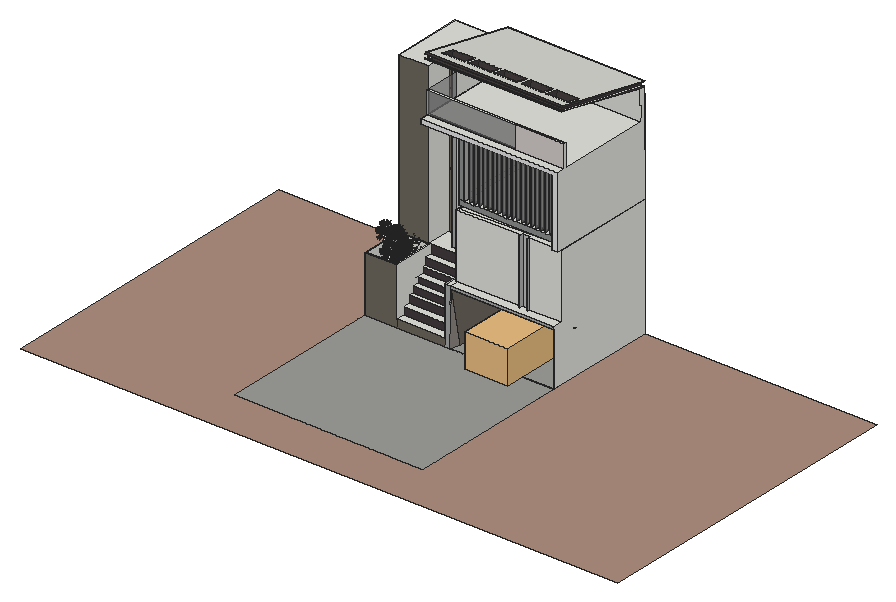
# SketchUp Ruby script. Lengths in inches.
U = 1.inch
M = Sketchup.active_model
def pt(a) = Geom::Point3d.new(a.map { |v| v * U })
def face(e, loops, mat)
  f = e.add_face(loops[0].map { |a| pt(a) })
  loops[1..].each { |l| e.add_face(l.map { |a| pt(a) }).erase! }
  f.material = f.back_material = mat if mat
  f
end
# faces: each face lists its corners as indices into pts; further lists are holes
def faces(e, pts, list, mat = nil) = list.each { |f| face(e, (f[0].is_a?(Array) ? f : [f]).map { |l| l.map { |i| pts[i] } }, mat) }
# xy, xz, yz: faces in a plane at the given z, y or x. An outline is a flat list of corners, or four numbers for a rectangle; further outlines are holes
def ring(l) = l.size == 4 ? [[l[0], l[1]], [l[2], l[1]], [l[2], l[3]], [l[0], l[3]]] : l.each_slice(2).to_a
def flat(e, list, mat, &to3) = list.each { |f| face(e, (f[0].is_a?(Array) ? f : [f]).map { |l| ring(l).map { |u, v| to3.(u, v) } }, mat) }
def xy(e, z, list, mat = nil) = flat(e, list, mat) { |x, y| [x, y, z] }
def xz(e, y, list, mat = nil) = flat(e, list, mat) { |x, z| [x, y, z] }
def yz(e, x, list, mat = nil) = flat(e, list, mat) { |y, z| [x, y, z] }
def lines(e, pts, list) = list.each { |a, b| e.add_line(pt(pts[a]), pt(pts[b])) }
# prism: a flat outline (further loops are holes) pulled along v
def prism(e, loops, v, mat = nil)
  f = face(e, loops, mat); d = Geom::Vector3d.new(v.map { |x| x * U })
  f.pushpull(f.normal.samedirection?(d) ? d.length : -d.length)
end
def box(e, o, s, mat = nil) = prism(e, [[o, [o[0] + s[0], o[1], o[2]], [o[0] + s[0], o[1] + s[1], o[2]], [o[0], o[1] + s[1], o[2]]]], [0, 0, s[2]], mat)
def at(x, y, z, deg = 0) = Geom::Transformation.translation(pt([x, y, z])) * Geom::Transformation.rotation(ORIGIN, Z_AXIS, deg.degrees)
def axes(o, x, y, z) = Geom::Transformation.new([*x, 0, *y, 0, *z, 0, *pt(o).to_a, 1])
def part(name) = M.definitions.add(name)
# library, detail: a bought-in or finely detailed component or shape, given as its bounding box
def library(name, o, s) = part(name).tap { |d| box(d.entities, o, s) }
def detail(e, o, s) = box(e.add_group.entities, o, s)
def put(e, d, t, mat = nil) = e.add_instance(d, t).tap { |i| i.material = mat if mat }
def group(e, t, mat = nil) = e.add_group.tap { |g| g.transformation = t; g.material = mat if mat }.entities
root = M.entities
M.materials.add("[Aluminum]").color = [179, 179, 179]
M.materials.add("[Asphalt New]").color = [67, 60, 62]
M.materials.add("[Blacktop Old 02]").color = [143, 145, 145]
M.materials.add("[Cladding Weathered]").color = [111, 105, 96]
M.materials.add("[Color M00]").color = [255, 255, 255]
M.materials.add("[Concrete Block 8x8 Gray]").color = [157, 158, 154]
M.materials.add("[Concrete Form 4x8]").color = [167, 170, 168]
M.materials.add("[Concrete Scored Jointless]").color = [140, 133, 127]
M.materials.add("[Metal Corrugated Shiny]").color = [193, 193, 193]
M.materials.add("[Pavers Modular Brick]").color = [175, 143, 129]
M.materials.add("[Polished Concrete Old]").color = [229, 229, 229]
M.materials.add("[Tile Hexagon White]").color = [213, 206, 204]
M.materials.add("[Translucent Glass Gray]").color = [128, 128, 128]
M.materials["[Translucent Glass Gray]"].alpha = 0.5
c1 = part("Group\#1")
xy(c1.entities,0,[[0.75,0,0.75,11.8125,1.49,9.04]])
p = [[0.75,11.8125,0],[0,8.59,0.28],[0.75,0,0]]
faces(c1.entities,p,[[0,1,2]])
c2 = part("Group\#2")
put(c2.entities,c1,axes([14.375,5.39,3.77],[0.45748,0.87256,0.17132],[-0.80767,0.48834,-0.33043],[-0.37199,0.0128,0.92815]))
put(c2.entities,c1,axes([-0.67,1.875,2.66],[0.89879,-0.42343,0.11346],[0.43837,0.86817,-0.23263],[0,0.25882,0.96593]))
put(c2.entities,c1,at(4.43,0,0))
c3 = part("Group\#11")
put(c3.entities,c2,axes([22.24,16.83,2.07],[-0.74431,0.66783,0],[-0.65748,-0.73278,-0.17537],[-0.11712,-0.13053,0.9845]))
put(c3.entities,c2,axes([5.44,0,2.07],[1,0,0],[0,0.9845,-0.17537],[0,0.17537,0.9845]))
put(c3.entities,c2,axes([11.93,24.29,2.07],[-0.95052,-0.31068,0],[0.30586,-0.93579,-0.17537],[0.05448,-0.16669,0.9845]))
c4 = part("Group\#4")
put(c4.entities,c3,axes([14.86,-1.73,0.2],[0.445,0.77076,0],[-0.77076,0.445,0],[0,0,1.5842]))
put(c4.entities,c3,at(0,0,0))
c5 = part("Group\#3")
put(c5.entities,c2,axes([22.24,16.83,2.07],[-0.74431,0.66783,0],[-0.65748,-0.73278,-0.17537],[-0.11712,-0.13053,0.9845]))
put(c5.entities,c2,axes([5.44,0,2.07],[1,0,0],[0,0.9845,-0.17537],[0,0.17537,0.9845]))
put(c5.entities,c2,axes([11.93,24.29,2.07],[-0.95052,-0.31068,0],[0.30586,-0.93579,-0.17537],[0.05448,-0.16669,0.9845]))
c6 = part("plant+06")
g1 = group(c6.entities,at(-18.2,-4.83,0,-28.132))
g2 = group(g1,at(16.21,1.96,0.15,45))
g3 = group(g2,at(0,13.2,6.74))
p = [[6.87,-6.88,6.35],[6.87,-6.88,1.06]]
lines(g3,p,[[0,1]])
put(g3,c3,axes([13.75,-0.59,5.87],[0,-0.5917,0],[-0.5917,0,0],[0,0,0.5917]))
put(g3,c3,axes([16.18,-7.3,4.96],[-0.4184,-0.4184,0],[-0.4184,0.4184,0],[0,0,0.39243]))
put(g3,c3,axes([7.21,-16.1875,5.36],[-0.45127,0.38271,0],[0.38271,0.45127,0],[0,0,0.5917]))
put(g3,c3,axes([9.38,1.03,7.16],[0.26331,-0.45606,0],[-0.45606,-0.26331,0],[0,0,0.93737]))
put(g3,c4,axes([11.69,-2.37,6.35],[0,-0.4246,0],[-0.41463,0,0],[0,0,0.79418]))
put(g3,c4,axes([13.04,-1.11,5.01],[0,-0.54349,0],[-0.53072,0,0],[0,0,-0.63534]))
g4 = group(g2,at(6.41,6.51,0))
yz(g4,0,[[2.84,0,3.35,0,3.59,0.57,3.4,0.57,3.35,1.6,2.95,3.43,2.26,4.68,1.45,5.78,0.57,8.92,0.06,13.45,0,8.85,0.92,5.52,1.78,4.37,2.41,3.22,2.78,1.53]])
g5 = group(g1,at(11.08,10.15,0))
p = [[0.67,0.67,15.45],[0.64,0.64,18.83],[1.01,1.01,27.22],[0.53,0.53,32.8],[0.79,0.79,27.32],[0.38,0.38,23.38],
  [0,0,18.98],[0.02,0.02,15.18],[1.0625,1.0625,8.07],[2,2,4.77],[2.6875,2.6875,0],[3.37,3.37,0],
  [3.15,3.15,1.52],[2.58,2.58,5.45],[1.65,1.65,8.75]]
faces(g5,p,[[0,1,2,3,4,5,6,7,8,9,10,11,12,13,14]])
g6 = group(g1,at(0,22.3,24.33))
p = [[11.61,-11.625,10.73],[11.61,-11.625,1.79]]
lines(g6,p,[[0,1]])
put(g6,c3,axes([23.24,-1,9.91],[0,-1,0],[-1,0,0],[0,0,1]))
put(g6,c3,axes([27.34,-12.34,8.39],[-0.70711,-0.70711,0],[-0.70711,0.70711,0],[0,0,0.66323]))
put(g6,c3,axes([12.1875,-27.36,9.06],[-0.76267,0.64679,0],[0.64679,0.76267,0],[0,0,1]))
put(g6,c5,axes([12.75,-8.02,11.21],[0.12015,-0.20811,0],[-0.20811,-0.12015,0],[0,0,2.51293]))
put(g6,c4,axes([19.76,-4,10.73],[0,-0.7176,0],[-0.70074,0,0],[0,0,1.3422]))
put(g6,c4,axes([22.04,-1.87,8.47],[0,-0.91853,0],[-0.89694,0,0],[0,0,-1.07376]))
g7 = group(g1,at(13.77,10.12,0.15))
yz(g7,0,[[3.35,0,3.86,0,5.625,2.125,6.92,4.34,7.79,6.82,9.06,9.4,9.5,10.42,9.57,11.59,9.18,14.18,9.77,19.63,8.6,14.17,8.89,11.53,8.79,10.51,8.36,9.61,6.96,7.04,6.47,5.81,6.17,4.6,5.15,2.46,3.59,0.57]])
g8 = group(g1,at(2.16,8.02,10.39))
p = [[11.61,11.625,10.73],[11.61,11.625,1.79]]
lines(g8,p,[[0,1]])
put(g8,c3,at(23.24,1,9.91,90))
put(g8,c3,axes([27.34,12.34,8.39],[-0.70711,0.70711,0],[-0.70711,-0.70711,0],[0,0,0.66323]))
put(g8,c3,at(12.1875,27.36,9.06,-139.7))
put(g8,c3,axes([15.85,-1.74,10.73],[0.445,0.77076,0],[-0.77076,0.445,0],[0,0,1.5842]))
put(g8,c4,axes([22.04,1.87,8.47],[0,0.91853,0],[-0.89694,0,0],[0,0,-1.07376]))
put(g8,c5,axes([12.75,15.23,10.63],[0.12015,-0.20811,0],[-0.20811,-0.12015,0],[0,0,2.11086]))
c7 = library("car\#1",[0.01,0.03,0.02],[18.76,39.97,12.32])
xy(root,0,[[256.5,66.7,532,304.75],[256.5,304.75,532,469.75]],"[Concrete Block 8x8 Gray]")
xy(root,0,[[0,0,0,469.75,256.5,469.75,256.5,66.7,532,66.7,532,469.75,868.5,469.75,868.5,0]],"[Pavers Modular Brick]")
xy(root,11.4375,[[303.32,304.75,373.81,317.05]])
xy(root,21.9375,[[303.32,317.05,373.81,327.17]])
xy(root,32.4375,[[303.32,327.17,373.81,333.97]])
xy(root,41.28,[[303.32,333.97,373.81,342.22]])
xy(root,50.125,[[303.32,342.22,373.81,352.48]])
xy(root,58.5625,[[303.32,352.48,373.81,356.36]])
xy(root,68.875,[[303.32,356.36,373.81,367.35]])
xy(root,77.99,[[383.9,304.75,528.81,468.375]],"[Concrete Scored Jointless]")
xy(root,81.1875,[[[256.5,304.75,303.32,367.35],[258.53,306.78,301.29,365.32]],[373.81,304.75,380.71,304.75,380.71,318.49,378.74,318.49,378.74,423.52,373.81,423.52],[380.71,304.75,532,304.75,532,318.49,484.37,318.49,484.37,315.8,483.53,315.8,483.53,320.92,473.54,320.92,473.54,315.8,472.125,315.8,472.125,318.49,380.71,318.49],[378.74,318.49,380.71,423.52],[299.38,367.35,373.81,367.35,373.81,423.52,332.89,423.52,332.89,377.29,325.25,377.29,325.25,403.55,299.38,403.55],
  [332.89,427.84,378.74,469.75]])
xy(root,103.5,[[336.62,423.34,338.18,427.84]],"[Translucent Glass Gray]")
xy(root,154.875,[[336.62,423.34,338.18,427.84]],"[Translucent Glass Gray]")
xy(root,174.1875,[[472.125,315.8,473.54,315.8,473.54,320.92,483.53,320.92,483.53,315.8,484.37,315.8,484.37,318.49,523.01,318.49,523.01,469.75,378.74,469.75,378.74,394.12,380.74,394.12,380.74,323.56,378.74,323.56,378.74,318.49,472.125,318.49],[523.01,318.49,532,469.75],[378.74,323.56,380.74,394.12]])
xy(root,175.74,[[523.01,311.36,532,469.75]])
xy(root,178.55,[[379.42,321.87,523.01,469.75]])
xy(root,186.36,[[387.1,321.87,388.32,328.37],[389.15,321.87,395.2,328.37],[396.02,321.87,402.07,328.37],[402.9,321.87,408.95,328.37],[409.77,321.87,415.82,328.37],
  [416.65,321.87,422.7,328.37],[423.52,321.87,429.57,328.37],[430.4,321.87,436.45,328.37],[437.27,321.87,443.32,328.37],[444.15,321.87,450.2,328.37],
  [451.02,321.87,457.07,328.37],[457.9,321.87,463.95,328.37],[464.77,321.87,470.82,328.37],[471.65,321.87,477.7,328.37],[478.52,321.87,484.57,328.37],
  [485.4,321.87,491.45,328.37],[492.27,321.87,498.32,328.37],[499.15,321.87,505.2,328.37],[506.02,321.87,512.07,328.37],[512.9,321.87,518.95,328.37],
  [519.77,321.87,523.01,328.37]])
xy(root,269.125,[[332.89,423.52,378.74,427.84]])
xy(root,270.4375,[[379.42,321.87,387.1,321.87,387.1,328.37,523.01,328.37,523.01,469.75,379.42,469.75],[388.32,321.87,389.15,328.37],[395.2,321.87,396.02,328.37],[402.07,321.87,402.9,328.37],[408.95,321.87,409.77,328.37],
  [415.82,321.87,416.65,328.37],[422.7,321.87,423.52,328.37],[429.57,321.87,430.4,328.37],[436.45,321.87,437.27,328.37],[443.32,321.87,444.15,328.37],
  [450.2,321.87,451.02,328.37],[457.07,321.87,457.9,328.37],[463.95,321.87,464.77,328.37],[470.82,321.87,471.65,328.37],[477.7,321.87,478.52,328.37],
  [484.57,321.87,485.4,328.37],[491.45,321.87,492.27,328.37],[498.32,321.87,499.15,328.37],[505.2,321.87,506.02,328.37],[512.07,321.87,512.9,328.37],
  [518.95,321.87,519.77,328.37]])
xy(root,272.72,[[332.89,311.36,523.01,469.75]])
xy(root,279.5,[[332.89,311.36,532,322.79],[332.89,325.46,532,461.81]])
xy(root,311.875,[[332.89,322.79,461.48,325.46],[461.48,322.79,532,325.46],[256.5,367.35,299.38,367.35,299.38,403.55,303.32,403.55,303.32,469.75,256.5,469.75],[325.25,377.29,332.89,469.75],[303.32,403.55,325.25,469.75]])
xy(root,323.37,[[332.89,467.54,339.64,467.82]])
xz(root,304.75,[[256.5,0,303.32,81.1875],[303.32,0,373.81,11.4375]],"[Cladding Weathered]")
xz(root,304.75,[[373.81,0,380.71,81.1875],[380.71,0,383.9,77.99,528.81,77.99,532,81.1875,380.71,81.1875]],"[Concrete Form 4x8]")
xz(root,306.78,[[258.53,63.625,301.29,81.1875]])
xz(root,311.36,[[523.01,175.74,532,175.74,532,279.5,332.89,279.5,332.89,272.72,523.01,272.72]],"[Polished Concrete Old]")
xz(root,315.8,[[472.125,81.1875,473.54,174.1875],[483.53,81.1875,484.37,174.1875]],"[Aluminum]")
xz(root,317.05,[[303.32,11.4375,373.81,21.9375]],"[Asphalt New]")
xz(root,318.42,[[332.89,354.89,532,356.22]],"[Asphalt New]")
xz(root,318.49,[[378.74,81.1875,472.125,174.1875],[484.37,81.1875,532,174.1875]])
xz(root,320.92,[[473.54,81.1875,483.53,174.1875]],"[Metal Corrugated Shiny]")
xz(root,321.87,[[379.42,178.55,523.01,178.55,523.01,186.36,519.77,186.36,519.77,270.4375,518.95,270.4375,518.95,186.36,512.9,186.36,512.9,270.4375,512.07,270.4375,512.07,186.36,506.02,186.36,506.02,270.4375,505.2,270.4375,505.2,186.36,499.15,186.36,499.15,270.4375,498.32,270.4375,498.32,186.36,492.27,186.36,492.27,270.4375,491.45,270.4375,491.45,186.36,485.4,186.36,485.4,270.4375,484.57,270.4375,484.57,186.36,478.52,186.36,478.52,270.4375,477.7,270.4375,477.7,186.36,471.65,186.36,471.65,270.4375,470.82,270.4375,470.82,186.36,464.77,186.36,464.77,270.4375,463.95,270.4375,463.95,186.36,457.9,186.36,457.9,270.4375,457.07,270.4375,457.07,186.36,451.02,186.36,451.02,270.4375,450.2,270.4375,450.2,186.36,444.15,186.36,444.15,270.4375,443.32,270.4375,443.32,186.36,437.27,186.36,437.27,270.4375,436.45,270.4375,436.45,186.36,430.4,186.36,430.4,270.4375,429.57,270.4375,429.57,186.36,423.52,186.36,423.52,270.4375,422.7,270.4375,422.7,186.36,416.65,186.36,416.65,270.4375,415.82,270.4375,415.82,186.36,409.77,186.36,409.77,270.4375,408.95,270.4375,408.95,186.36,402.9,186.36,402.9,270.4375,402.07,270.4375,402.07,186.36,396.02,186.36,396.02,270.4375,395.2,270.4375,395.2,186.36,389.15,186.36,389.15,270.4375,388.32,270.4375,388.32,186.36,379.42,186.36],[379.42,186.36,387.1,270.4375]],"[Blacktop Old 02]")
xz(root,322.79,[[461.48,279.5,532,311.875]],"[Tile Hexagon White]")
xz(root,322.79,[[332.89,279.5,461.48,311.875]],"[Translucent Glass Gray]")
xz(root,325.46,[[461.48,279.5,532,311.875]])
xz(root,325.46,[[332.89,279.5,461.48,311.875]],"[Translucent Glass Gray]")
xz(root,327.17,[[303.32,21.9375,373.81,32.4375]],"[Asphalt New]")
xz(root,328.37,[[387.1,186.36,388.32,270.4375]])
xz(root,328.37,[[389.15,186.36,395.2,270.4375],[396.02,186.36,402.07,270.4375],[402.9,186.36,408.95,270.4375],[409.77,186.36,415.82,270.4375],[416.65,186.36,422.7,270.4375],
  [423.52,186.36,429.57,270.4375],[430.4,186.36,436.45,270.4375],[437.27,186.36,443.32,270.4375],[444.15,186.36,450.2,270.4375],[451.02,186.36,457.07,270.4375],
  [457.9,186.36,463.95,270.4375],[464.77,186.36,470.82,270.4375],[471.65,186.36,477.7,270.4375],[478.52,186.36,484.57,270.4375],[485.4,186.36,491.45,270.4375],
  [492.27,186.36,498.32,270.4375],[499.15,186.36,505.2,270.4375],[506.02,186.36,512.07,270.4375],[512.9,186.36,518.95,270.4375],[519.77,186.36,523.01,270.4375]],"[Translucent Glass Gray]")
xz(root,333.97,[[303.32,32.4375,373.81,41.28]],"[Asphalt New]")
xz(root,342.22,[[303.32,41.28,373.81,50.125]],"[Asphalt New]")
xz(root,352.48,[[303.32,50.125,373.81,58.5625]],"[Asphalt New]")
xz(root,356.36,[[303.32,58.5625,373.81,68.875]],"[Asphalt New]")
xz(root,365.32,[[258.53,63.625,299.38,81.1875]])
xz(root,367.35,[[303.32,68.875,373.81,81.1875]],"[Asphalt New]")
xz(root,367.35,[[256.5,81.1875,299.38,311.875]],"[Cladding Weathered]")
xz(root,377.29,[[325.25,81.1875,332.89,311.875]],"[Concrete Form 4x8]")
xz(root,403.55,[[[302.32,122.77,325.25,299.71],[303.625,124.08,323.94,298.4]],[303.625,163.67,323.94,165.07],[303.625,219.03,323.94,220.97],[303.625,268.56,323.94,270.61]],"[Asphalt New]")
xz(root,403.55,[[299.38,81.1875,325.25,81.1875,325.25,122.77,302.32,122.77,302.32,299.71,325.25,299.71,325.25,311.875,299.38,311.875]],"[Cladding Weathered]")
xz(root,423.34,[[336.62,103.5,338.18,154.875]],"[Translucent Glass Gray]")
xz(root,423.52,[[332.89,177.19,378.74,180.2]],"[Asphalt New]")
xz(root,423.52,[[332.89,81.1875,378.74,177.19]],"[Translucent Glass Gray]")
xz(root,427.84,[[[332.89,81.1875,378.74,269.125],[336.62,103.5,338.18,154.875]]],"[Translucent Glass Gray]")
xz(root,468.375,[[383.9,3.19,528.81,77.99]],"[Cladding Weathered]")
xz(root,469.75,[[332.89,81.1875,378.74,272.72],[378.74,174.1875,378.74,272.72,523.01,272.72,523.01,270.4375,379.42,270.4375,379.42,178.55,380.74,178.55,380.74,174.1875],[380.74,174.1875,523.01,178.55],[523.01,174.1875,532,175.74],[523.01,175.74,523.01,178.55,379.42,178.55,379.42,270.4375,523.01,270.4375,523.01,182.6875,532,182.6875,532,175.74],
  [532,182.6875,523.01,270.4375,523.01,272.72,332.89,311.875,532,311.875],[523.01,182.6875,523.01,270.4375,532,182.6875],[332.89,272.72,332.89,311.875,523.01,272.72]])
xz(root,469.75,[[256.5,0,332.89,311.875],[332.89,0,332.89,81.1875,378.74,81.1875,378.74,174.1875,532,174.1875,532,0]],"[Color M00]")
yz(root,256.5,[[304.75,0,304.75,81.1875,367.35,81.1875,367.35,311.875,469.75,311.875,469.75,0]])
yz(root,258.53,[[306.78,63.625,365.32,81.1875]])
yz(root,299.38,[[367.35,81.1875,403.55,311.875]])
yz(root,303.32,[[304.75,11.4375,317.05,11.4375,317.05,21.9375,327.17,21.9375,327.17,32.4375,333.97,32.4375,333.97,41.28,342.22,41.28,342.22,50.125,352.48,50.125,352.48,58.5625,356.36,58.5625,356.36,68.875,367.35,68.875,367.35,81.1875,304.75,81.1875]])
yz(root,325.25,[[377.29,81.1875,403.55,311.875]])
yz(root,332.89,[[377.29,81.1875,423.52,81.1875,423.52,269.125,427.84,269.125,427.84,81.1875,469.75,81.1875,469.75,272.72,377.29,272.72],[311.36,272.72,377.29,279.5],[377.29,272.72,377.29,279.5,461.81,279.5,461.81,311.875,469.75,311.875,469.75,272.72],[322.79,279.5,325.46,311.875],[377.29,279.5,461.81,279.5,460.34,311.875,377.29,311.875],
  [461.81,279.5,461.81,311.875,460.34,311.875],[460.34,311.875,459.79,323.81,461.81,311.875],[461.81,311.875,459.79,323.81,467.54,322.11,469.75,311.875]])
yz(root,332.89,[[467.54,322.11,459.79,323.81,323.42,353.79,323.6875,355,467.54,323.37,467.82,323.37],[468.8,327.8125,324.68,359.5,319.67,360.6,320.06,362.35,469.18,329.5625]],"[Asphalt New]")
yz(root,332.89,[[325.46,279.5,377.29,311.875]],"[Translucent Glass Gray]")
yz(root,336.62,[[423.34,103.5,427.84,154.875]],"[Translucent Glass Gray]")
yz(root,338.18,[[423.34,103.5,427.84,154.875]],"[Translucent Glass Gray]")
yz(root,339.64,[[467.54,323.37,323.6875,355,324.68,359.5,468.8,327.8125,467.82,323.37]],"[Asphalt New]")
yz(root,344.65,[[353.31,347.22,354.95,354.68,335.23,359.01,333.59,351.56]],"[Asphalt New]")
yz(root,373.81,[[304.75,11.4375,304.75,81.1875,367.35,81.1875,367.35,68.875,356.36,68.875,356.36,58.5625,352.48,58.5625,352.48,50.125,342.22,50.125,342.22,41.28,333.97,41.28,333.97,32.4375,327.17,32.4375,327.17,21.9375,317.05,21.9375,317.05,11.4375]])
yz(root,377.31,[[353.31,347.22,333.59,351.56,335.23,359.01,354.95,354.68]])
yz(root,378.74,[[318.49,81.1875,423.52,174.1875],[427.84,81.1875,469.75,174.1875],[423.52,174.1875,427.84,269.125]])
yz(root,379.42,[[321.87,178.55,469.75,186.36],[321.87,186.36,469.75,270.4375]])
yz(root,382.28,[[353.31,347.22,354.95,354.68,335.23,359.01,333.59,351.56]],"[Asphalt New]")
yz(root,383.9,[[322.9,-14.85,468.375,3.19,468.375,77.99,304.75,77.99,468.375,3.82],[322.9,-14.85,468.375,3.82,304.75,77.99]],"[Cladding Weathered]")
yz(root,387.1,[[321.87,186.36,328.37,270.4375]])
yz(root,388.32,[[321.87,186.36,328.37,270.4375]])
yz(root,389.15,[[321.87,186.36,328.37,270.4375]],"[Translucent Glass Gray]")
yz(root,395.2,[[321.87,186.36,328.37,270.4375]],"[Translucent Glass Gray]")
yz(root,396.02,[[321.87,186.36,328.37,270.4375]],"[Translucent Glass Gray]")
yz(root,402.07,[[321.87,186.36,328.37,270.4375]],"[Translucent Glass Gray]")
yz(root,402.9,[[321.87,186.36,328.37,270.4375]],"[Translucent Glass Gray]")
yz(root,408.95,[[321.87,186.36,328.37,270.4375]],"[Translucent Glass Gray]")
yz(root,409.77,[[321.87,186.36,328.37,270.4375]],"[Translucent Glass Gray]")
yz(root,414.94,[[353.31,347.22,333.59,351.56,335.23,359.01,354.95,354.68]])
yz(root,415.82,[[321.87,186.36,328.37,270.4375]],"[Translucent Glass Gray]")
yz(root,416.65,[[321.87,186.36,328.37,270.4375]],"[Translucent Glass Gray]")
yz(root,420.09,[[353.31,347.22,354.95,354.68,335.23,359.01,333.59,351.56]],"[Asphalt New]")
yz(root,422.7,[[321.87,186.36,328.37,270.4375]],"[Translucent Glass Gray]")
yz(root,423.52,[[321.87,186.36,328.37,270.4375]],"[Translucent Glass Gray]")
yz(root,429.57,[[321.87,186.36,328.37,270.4375]],"[Translucent Glass Gray]")
yz(root,430.4,[[321.87,186.36,328.37,270.4375]],"[Translucent Glass Gray]")
yz(root,436.45,[[321.87,186.36,328.37,270.4375]],"[Translucent Glass Gray]")
yz(root,437.27,[[321.87,186.36,328.37,270.4375]],"[Translucent Glass Gray]")
yz(root,443.32,[[321.87,186.36,328.37,270.4375]],"[Translucent Glass Gray]")
yz(root,444.15,[[321.87,186.36,328.37,270.4375]],"[Translucent Glass Gray]")
yz(root,450.2,[[321.87,186.36,328.37,270.4375]],"[Translucent Glass Gray]")
yz(root,451.02,[[321.87,186.36,328.37,270.4375]],"[Translucent Glass Gray]")
yz(root,452.75,[[353.31,347.22,333.59,351.56,335.23,359.01,354.95,354.68]])
yz(root,457.07,[[321.87,186.36,328.37,270.4375]],"[Translucent Glass Gray]")
yz(root,457.9,[[321.87,186.36,328.37,270.4375]],"[Translucent Glass Gray]")
yz(root,458.15,[[353.31,347.22,354.95,354.68,335.23,359.01,333.59,351.56]],"[Asphalt New]")
yz(root,463.95,[[321.87,186.36,328.37,270.4375]],"[Translucent Glass Gray]")
yz(root,464.77,[[321.87,186.36,328.37,270.4375]],"[Translucent Glass Gray]")
yz(root,470.82,[[321.87,186.36,328.37,270.4375]],"[Translucent Glass Gray]")
yz(root,471.65,[[321.87,186.36,328.37,270.4375]],"[Translucent Glass Gray]")
yz(root,472.125,[[315.8,81.1875,318.49,174.1875]],"[Aluminum]")
yz(root,473.54,[[315.8,81.1875,320.92,174.1875]],"[Aluminum]")
yz(root,477.7,[[321.87,186.36,328.37,270.4375]],"[Translucent Glass Gray]")
yz(root,478.52,[[321.87,186.36,328.37,270.4375]],"[Translucent Glass Gray]")
yz(root,483.53,[[315.8,81.1875,320.92,174.1875]],"[Aluminum]")
yz(root,484.37,[[315.8,81.1875,318.49,174.1875]],"[Aluminum]")
yz(root,484.57,[[321.87,186.36,328.37,270.4375]],"[Translucent Glass Gray]")
yz(root,485.4,[[321.87,186.36,328.37,270.4375]],"[Translucent Glass Gray]")
yz(root,490.81,[[353.31,347.22,333.59,351.56,335.23,359.01,354.95,354.68]])
yz(root,491.45,[[321.87,186.36,328.37,270.4375]],"[Translucent Glass Gray]")
yz(root,492.27,[[321.87,186.36,328.37,270.4375]],"[Translucent Glass Gray]")
yz(root,495.65,[[353.31,347.22,354.95,354.68,335.23,359.01,333.59,351.56]],"[Asphalt New]")
yz(root,498.32,[[321.87,186.36,328.37,270.4375]],"[Translucent Glass Gray]")
yz(root,499.15,[[321.87,186.36,328.37,270.4375]],"[Translucent Glass Gray]")
yz(root,505.2,[[321.87,186.36,328.37,270.4375]],"[Translucent Glass Gray]")
yz(root,506.02,[[321.87,186.36,328.37,270.4375]],"[Translucent Glass Gray]")
yz(root,512.07,[[321.87,186.36,328.37,270.4375]],"[Translucent Glass Gray]")
yz(root,512.9,[[321.87,186.36,328.37,270.4375]],"[Translucent Glass Gray]")
yz(root,518.95,[[321.87,186.36,328.37,270.4375]],"[Translucent Glass Gray]")
yz(root,519.77,[[321.87,186.36,328.37,270.4375]])
yz(root,523.01,[[311.36,175.74,311.36,272.72,469.75,272.72,469.75,270.4375,328.37,270.4375,328.37,186.36,321.87,186.36,321.87,178.55,323.56,178.55,323.56,175.74],[323.56,175.74,469.75,178.55]])
yz(root,528.3125,[[353.31,347.22,333.59,351.56,333.83,352.65,353.55,348.3125],[354.5625,352.93,334.84,357.26,335.23,359.01,354.95,354.68]])
yz(root,528.3125,[[467.78,323.2,468.8,327.8125,354.5625,352.93,353.55,348.3125],[353.55,348.3125,354.5625,352.93,334.84,357.26,333.83,352.65],[333.83,352.65,334.84,357.26,324.68,359.5,323.66,354.88]],"[Asphalt New]")
yz(root,528.81,[[322.9,-14.85,468.375,3.82,304.75,77.99,468.375,77.99,468.375,3.19]],"[Cladding Weathered]")
yz(root,532,[[304.75,0,469.75,0,469.75,174.1875,318.49,174.1875,318.49,81.1875,304.75,81.1875],[311.36,175.74,469.75,175.74,469.75,182.6875,467.54,322.11,459.79,323.81,461.81,279.5,325.46,279.5,325.46,311.875,322.79,311.875,322.79,279.5,311.36,279.5]])
yz(root,532,[[467.54,322.11,467.78,323.2,323.66,354.88,323.42,353.79,459.79,323.81],[468.8,327.8125,469.18,329.5625,320.06,362.35,319.67,360.6,324.68,359.5]],"[Asphalt New]")
p = [[532,304.75,0],[380.71,304.75,0],[383.9,322.9,-14.85],[528.81,322.9,-14.85],[383.9,304.75,77.99],[532,304.75,81.1875],
  [528.81,468.375,3.82],[383.9,468.375,3.19],[528.81,468.375,3.19],[528.81,304.75,77.99],[380.74,323.56,174.1875],[523.01,323.56,178.55],
  [523.01,394.12,178.55],[380.74,394.12,174.1875],[532,467.54,322.11],[532,469.75,182.6875],[523.01,469.75,270.4375],[523.01,469.75,272.72],
  [332.89,469.75,311.875],[532,461.81,279.5],[532,459.79,323.81],[332.89,461.81,279.5],[332.89,461.81,311.875],[332.89,460.34,311.875],
  [528.3125,459.79,323.81],[343.45,459.79,323.81],[332.89,459.79,323.81],[332.89,467.54,322.11],[532,467.78,323.2],[332.89,467.82,323.37],
  [339.64,467.82,323.37],[339.64,468.8,327.8125],[332.89,468.8,327.8125],[332.89,469.18,329.5625],[532,469.18,329.5625],[532,468.8,327.8125],
  [528.3125,468.8,327.8125],[528.3125,467.78,323.2],[532,323.66,354.88],[528.3125,353.55,348.3125],[528.3125,333.83,352.65],[528.3125,323.66,354.88],
  [332.89,467.54,323.37],[332.89,323.6875,355],[339.64,323.6875,355],[339.64,467.54,323.37],[343.45,323.42,353.79],[332.89,323.42,353.79],
  [495.65,333.59,351.56],[528.3125,333.59,351.56],[528.3125,323.42,353.79],[528.3125,353.31,347.22],[495.65,353.31,347.22],[377.31,333.59,351.56],
  [377.31,353.31,347.22],[344.65,353.31,347.22],[344.65,333.59,351.56],[420.09,333.59,351.56],[452.75,333.59,351.56],[452.75,353.31,347.22],
  [420.09,353.31,347.22],[490.81,333.59,351.56],[490.81,353.31,347.22],[458.15,353.31,347.22],[458.15,333.59,351.56],[414.94,333.59,351.56],
  [414.94,353.31,347.22],[382.28,353.31,347.22],[382.28,333.59,351.56],[532,323.42,353.79],[332.89,324.68,359.5],[339.64,324.68,359.5],
  [532,324.68,359.5],[528.3125,324.68,359.5],[528.3125,334.84,357.26],[528.3125,354.5625,352.93],[332.89,320.06,362.35],[532,320.06,362.35],
  [377.31,354.95,354.68],[377.31,335.23,359.01],[344.65,335.23,359.01],[344.65,354.95,354.68],[414.94,354.95,354.68],[414.94,335.23,359.01],
  [382.28,335.23,359.01],[382.28,354.95,354.68],[452.75,335.23,359.01],[420.09,335.23,359.01],[420.09,354.95,354.68],[452.75,354.95,354.68],
  [490.81,354.95,354.68],[490.81,335.23,359.01],[458.15,335.23,359.01],[458.15,354.95,354.68],[528.3125,335.23,359.01],[495.65,335.23,359.01],
  [495.65,354.95,354.68],[528.3125,354.95,354.68],[532,318.42,354.89],[332.89,318.42,354.89],[532,319.67,360.6],[332.89,319.67,360.6],
  [526.65,328.37,186.36],[526.65,321.87,186.36],[525.82,321.87,186.36],[525.82,328.37,186.36],[683.43,3420.28,-738],[675.53,3431,-738],
  [301.29,365.32,63.625],[299.38,365.32,63.625],[373.81,321.92,32.4375],[373.81,327.17,32.4375],[303.32,339.1,50.125],[303.32,342.22,50.125],
  [373.81,339.1,50.125],[373.81,342.22,50.125]]
faces(root,p,[[0,1,2,3],[0,5,3],[9,6,5],[10,11,12,13],[14,15,16],[17,14,16],[18,14,17],[19,20,21],
  [22,21,20],[23,21,20,24,25,26],[26,22,20,24,25],[27,14,18],[27,14,20,24,25,26],[28,14,27,29,30,31,32,33,34,35,36,37],[38,28,37,39,40,41],[42,43,44,45],
  [[48,49,50,46,25,24,51,52],[53,54,55,56],[57,58,59,60],[61,62,63,64],[65,66,67,68]],[70,32,31,71],[[33,76,77,34],[78,79,80,81],[82,83,84,85],[86,87,88,89],[90,91,92,93],[94,95,96,97]],[80,79,53,56],[84,83,65,68],[87,86,58,57],[92,91,61,64],[95,94,74,40,49,48]])
faces(root,p,[[1,2,4]],"[Concrete Scored Jointless]")
faces(root,p,[[3,5,6]],"[Cladding Weathered]")
faces(root,p,[[7,8,3,2]],"[Concrete Block 8x8 Gray]")
faces(root,p,[[26,25,46,47],[69,50,49,51,24,20],[35,72,73,74,75,36],[78,81,55,54],[82,85,67,66],[89,88,60,59],[90,93,63,62],[97,96,52,51,39,75],
  [98,99,47,46,50,69],[69,38,41,73,71,44,43,47,46,50],[100,101,70,71,73,72],[76,101,100,77]],"[Asphalt New]")
lines(root,p,[[102,103],[104,105],[106,107],[108,109],[110,111],[112,113],[114,115]])
put(root,c6,at(278.9375,340.78,59.9375))
put(root,c6,at(261.65,340.78,59.9375))
put(root,c6,at(282.65,330.49,54.79))
put(root,c6,at(285.1,318.66,50.17))
put(root,c6,at(274.9,337.87,42.87))
put(root,c6,at(286.72,371.6875,40.1))
put(root,c7,axes([423.43,277.87,-0.07],[3.35,0,0],[0,4.02,0],[0,0,3.953]))
